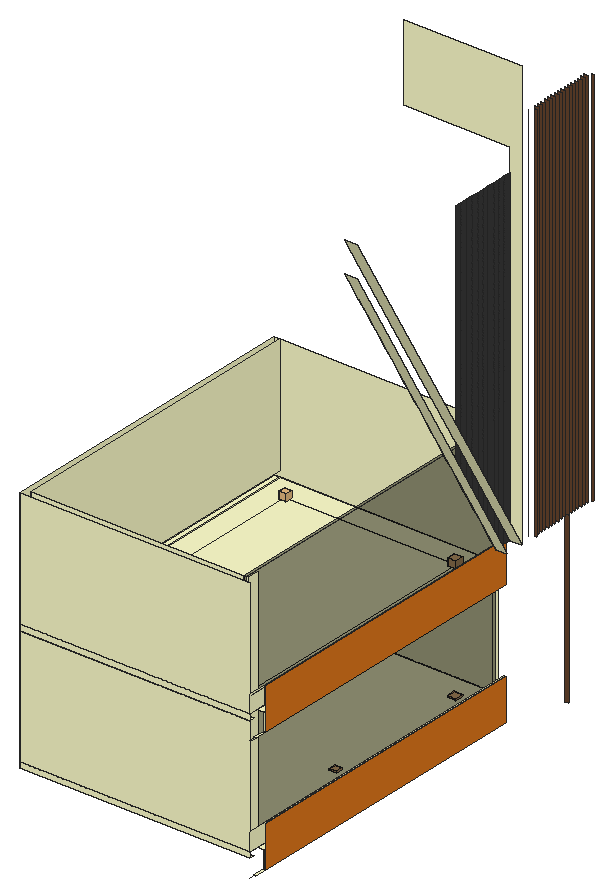
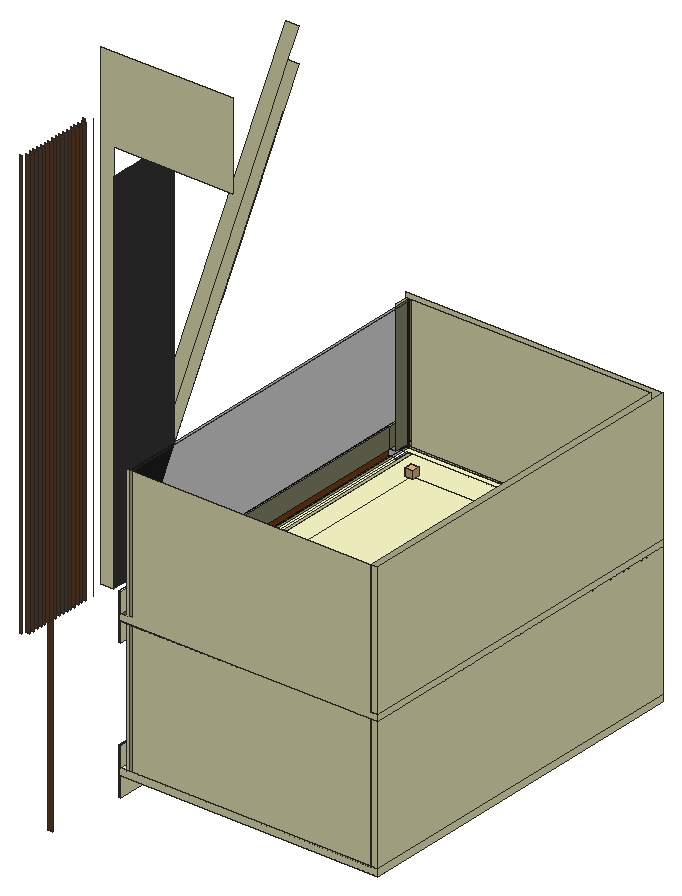
# SketchUp Ruby script. Lengths in inches.
U = 1.inch
M = Sketchup.active_model
def pt(a) = Geom::Point3d.new(a.map { |v| v * U })
def face(e, loops, mat)
  f = e.add_face(loops[0].map { |a| pt(a) })
  loops[1..].each { |l| e.add_face(l.map { |a| pt(a) }).erase! }
  f.material = f.back_material = mat if mat
  f
end
# faces: each face lists its corners as indices into pts; further lists are holes
def faces(e, pts, list, mat = nil) = list.each { |f| face(e, (f[0].is_a?(Array) ? f : [f]).map { |l| l.map { |i| pts[i] } }, mat) }
# xy, xz, yz: faces in a plane at the given z, y or x. An outline is a flat list of corners, or four numbers for a rectangle; further outlines are holes
def ring(l) = l.size == 4 ? [[l[0], l[1]], [l[2], l[1]], [l[2], l[3]], [l[0], l[3]]] : l.each_slice(2).to_a
def flat(e, list, mat, &to3) = list.each { |f| face(e, (f[0].is_a?(Array) ? f : [f]).map { |l| ring(l).map { |u, v| to3.(u, v) } }, mat) }
def xy(e, z, list, mat = nil) = flat(e, list, mat) { |x, y| [x, y, z] }
def xz(e, y, list, mat = nil) = flat(e, list, mat) { |x, z| [x, y, z] }
def yz(e, x, list, mat = nil) = flat(e, list, mat) { |y, z| [x, y, z] }
def lines(e, pts, list) = list.each { |a, b| e.add_line(pt(pts[a]), pt(pts[b])) }
# prism: a flat outline (further loops are holes) pulled along v
def prism(e, loops, v, mat = nil)
  f = face(e, loops, mat); d = Geom::Vector3d.new(v.map { |x| x * U })
  f.pushpull(f.normal.samedirection?(d) ? d.length : -d.length)
end
def box(e, o, s, mat = nil) = prism(e, [[o, [o[0] + s[0], o[1], o[2]], [o[0] + s[0], o[1] + s[1], o[2]], [o[0], o[1] + s[1], o[2]]]], [0, 0, s[2]], mat)
def at(x, y, z, deg = 0) = Geom::Transformation.translation(pt([x, y, z])) * Geom::Transformation.rotation(ORIGIN, Z_AXIS, deg.degrees)
def axes(o, x, y, z) = Geom::Transformation.new([*x, 0, *y, 0, *z, 0, *pt(o).to_a, 1])
def part(name) = M.definitions.add(name)
# library, detail: a bought-in or finely detailed component or shape, given as its bounding box
def library(name, o, s) = part(name).tap { |d| box(d.entities, o, s) }
def detail(e, o, s) = box(e.add_group.entities, o, s)
def put(e, d, t, mat = nil) = e.add_instance(d, t).tap { |i| i.material = mat if mat }
def group(e, t, mat = nil) = e.add_group.tap { |g| g.transformation = t; g.material = mat if mat }.entities
root = M.entities
M.materials.add("Brick_Common_Bond_2K").color = [226, 121, 29]
M.materials.add("E01_Mint_Frost").color = [255, 255, 204]
M.materials.add("Glass_Safety_01").color = [0, 0, 0]
M.materials["Glass_Safety_01"].alpha = 0.25
M.materials.add("M07_Charcoal_Gleam").color = [58, 58, 58]
M.materials.add("Wood_Veneer_15_1K").color = [103, 69, 45]
c1 = library("Sphere Light\#7",[-4.28,-4.28,-4.28],[8.56,8.56,8.56])
c2 = library("Sphere Light\#5",[-3.78,-3.78,-3.78],[7.56,7.56,7.56])
c3 = library("Sphere Light\#6",[-3.67,-3.67,-3.67],[7.34,7.34,7.34])
c4 = library("Sphere Light\#4",[-3.65,-3.65,-3.65],[7.3,7.3,7.3])
c5 = part("Group\#3")
box(c5.entities,[0,0,0],[3,318,120])
xy(root,240,[[469.07,81.71,471.07,93.71],[469.07,93.71,471.07,399.71]],"E01_Mint_Frost")
xy(root,258,[[235.07,75.71,469.07,81.71],[235.07,81.71,241.07,399.71],[[241.07,81.71,463.07,399.71],[439.07,101.71,440.11,101.85,441.07,102.25,441.9,102.89,442.54,103.71,442.9375,104.68,443.07,105.71,442.9375,106.75,442.54,107.71,441.9,108.54,441.07,109.18,440.11,109.58,439.07,109.71,439.07,371.72,440.02,371.83,441,372.21,441.84,372.82,442.49,373.64,442.91,374.59,443.07,375.625,442.96,376.66,442.58,377.64,441.96,378.48,441.15,379.13,440.19,379.55,439.16,379.71,438.125,379.6,437.15,379.22,436.31,378.6,435.65,377.79,435.23,376.83,435.07,375.8,435.08,375.71,269.05,375.71,269.0625,375.99,268.86,377.01,268.39,377.95,267.7,378.73,266.83,379.31,265.84,379.64,264.8,379.7,263.78,379.5,262.84,379.03,262.06,378.34,261.48,377.47,261.15,376.48,261.08,375.44,261.29,374.42,261.76,373.48,262.45,372.7,263.32,372.12,264.31,371.79,265.07,371.74,265.07,109.7,264.1875,109.61,263.21,109.25,262.35,108.65,261.6875,107.84,261.25,106.9,261.08,105.87,261.17,104.83,261.54,103.85,262.14,103,262.94,102.33,263.89,101.89,264.92,101.72,265.96,101.8125,266.94,102.18,267.79,102.78,268.46,103.58,268.9,104.53,269.07,105.5625,269.06,105.71,435.07,105.71,435.21,104.68,435.61,103.71,436.25,102.89,437.07,102.25,438.04,101.85]],[463.07,93.71,469.07,399.71],[269.06,105.71,268.97,106.6,268.61,107.58,268.01,108.43,267.2,109.1,266.25,109.54,265.23,109.71,265.07,109.7,265.07,371.74,265.35,371.72,266.37,371.93,267.31,372.4,268.09,373.09,268.67,373.96,269,374.95,269.05,375.71,435.08,375.71,435.1875,374.76,435.57,373.79,436.18,372.95,437,372.29,437.95,371.875,438.99,371.72,439.07,371.72,439.07,109.71,438.04,109.58,437.07,109.18,436.25,108.54,435.61,107.71,435.21,106.75,435.07,105.71]],"E01_Mint_Frost")
xy(root,261,[[439.07,101.71,438.04,101.85,437.07,102.25,436.25,102.89,435.61,103.71,435.21,104.68,435.07,105.71,435.21,106.75,435.61,107.71,436.25,108.54,437.07,109.18,438.04,109.58,439.07,109.71,440.11,109.58,441.07,109.18,441.9,108.54,442.54,107.71,442.9375,106.75,443.07,105.71,442.9375,104.68,442.54,103.71,441.9,102.89,441.07,102.25,440.11,101.85],[264.92,101.72,264.8,101.74,265.32,101.75],[264.8,101.74,264.29,101.83,263.78,101.94,263.31,102.16,262.85,102.41,262.45,102.74,262.07,103.1,261.77,103.52,261.49,103.96,261.3125,104.45,261.16,104.95,261.11,105.47,261.1,105.99,261.19,106.5,261.3,107.01,261.52,107.48,261.77,107.94,262.1,108.34,262.46,108.72,262.88,109.02,263.32,109.3,263.8125,109.48,264.3125,109.625,264.83,109.67,265.07,109.7,265.23,109.71,266.25,109.54,267.2,109.1,268.01,108.43,268.61,107.58,268.97,106.6,269.06,105.71,269.07,105.5625,269.05,105.4375,268.96,104.93,268.84,104.42,268.625,103.95,268.38,103.49,268.05,103.09,267.69,102.71,267.27,102.41,266.82,102.13,266.34,101.95,265.84,101.8,265.32,101.75],[265.84,101.8,266.34,101.95,265.96,101.8125],[264.29,101.83,263.89,101.89,263.78,101.94],
  [266.82,102.13,267.27,102.41,266.94,102.18],[263.31,102.16,262.94,102.33,262.85,102.41],[267.69,102.71,268.05,103.09,267.79,102.78],[262.45,102.74,262.14,103,262.07,103.1],[268.38,103.49,268.625,103.95,268.46,103.58],
  [261.77,103.52,261.54,103.85,261.49,103.96],[268.84,104.42,268.96,104.93,268.9,104.53],[261.3125,104.45,261.17,104.83,261.16,104.95],[261.11,105.47,261.08,105.87,261.1,105.99],[261.19,106.5,261.25,106.9,261.3,107.01],
  [261.52,107.48,261.6875,107.84,261.77,107.94],[262.1,108.34,262.35,108.65,262.46,108.72],[262.88,109.02,263.21,109.25,263.32,109.3],[263.8125,109.48,264.1875,109.61,264.3125,109.625],[265.35,371.72,265.07,371.74,264.31,371.79,263.32,372.12,262.45,372.7,261.76,373.48,261.29,374.42,261.08,375.44,261.15,376.48,261.48,377.47,262.06,378.34,262.84,379.03,263.78,379.5,264.8,379.7,265.84,379.64,266.83,379.31,267.7,378.73,268.39,377.95,268.86,377.01,269.0625,375.99,269.05,375.71,269,374.95,268.67,373.96,268.09,373.09,267.31,372.4,266.37,371.93],
  [438.99,371.72,437.95,371.875,437,372.29,436.18,372.95,435.57,373.79,435.1875,374.76,435.08,375.71,435.07,375.8,435.23,376.83,435.65,377.79,436.31,378.6,437.15,379.22,438.125,379.6,439.16,379.71,440.19,379.55,441.15,379.13,441.96,378.48,442.58,377.64,442.96,376.66,443.07,375.625,442.91,374.59,442.49,373.64,441.84,372.82,441,372.21,440.02,371.83,439.07,371.72]],"E01_Mint_Frost")
xy(root,264,[[235.07,75.71,469.07,75.71,469.07,93.71,463.07,93.71,463.07,81.71,241.07,81.71,241.07,399.71,235.07,399.71],[241.07,81.71,463.07,81.71,463.07,93.71,469.07,93.71,469.07,399.71,241.07,399.71]],"E01_Mint_Frost")
xy(root,282,[[469.07,93.71,471.07,399.71]],"E01_Mint_Frost")
xy(root,366,[[469.07,81.71,471.07,93.71],[469.07,93.71,471.07,399.71]],"E01_Mint_Frost")
xy(root,384,[[235.07,75.71,469.07,81.71],[235.07,81.71,241.07,399.71],[[241.07,81.71,463.07,399.71],[265.07,105.71,439.07,375.71]],[463.07,93.71,469.07,399.71],[265.07,105.71,439.07,375.71]],"E01_Mint_Frost")
xy(root,390,[[235.07,75.71,469.07,75.71,469.07,93.71,463.07,93.71,463.07,81.71,241.07,81.71,241.07,399.71,235.07,399.71]],"E01_Mint_Frost")
xy(root,408,[[469.07,93.71,471.07,399.71]],"E01_Mint_Frost")
xz(root,75.71,[[235.07,258,469.07,264],[235.07,264,469.07,384],[235.07,384,469.07,390],[235.07,390,469.07,510]],"E01_Mint_Frost")
xz(root,81.71,[[241.07,264,458.07,384],[461.07,264,463.07,384],[241.07,390,458.07,510],[461.07,390,463.07,510]],"E01_Mint_Frost")
xz(root,93.71,[[469.07,240,471.07,258]],"E01_Mint_Frost")
xz(root,371.72,[[438.99,258,439.07,261]],"E01_Mint_Frost")
xz(root,399.71,[[469.07,240,471.07,258],[235.07,258,471.07,264],[235.07,264,241.07,384],[241.07,264,463.07,384],[469.07,264,471.07,282],
  [469.07,366,471.07,384],[235.07,384,471.07,384,471.07,390,463.07,390,463.07,510,241.07,510,241.07,390,235.07,390],[235.07,390,241.07,510],[469.07,390,471.07,408],[475.07,408,487.07,408,487.07,846,367.07,846,367.07,768,475.07,768]],"E01_Mint_Frost")
xz(root,420,[[485.07,406.83,487.07,796.83]],"Wood_Veneer_15_1K")
xz(root,424.21,[[481.07,406.9,485.07,796.9]],"Wood_Veneer_15_1K")
xz(root,428.43,[[481.07,406.96,485.07,796.96]],"Wood_Veneer_15_1K")
xz(root,432.64,[[481.07,407.03,485.07,797.03]],"Wood_Veneer_15_1K")
xz(root,436.86,[[481.07,407.09,485.07,797.09]],"Wood_Veneer_15_1K")
xz(root,441.07,[[481.07,407.16,485.07,797.16]],"Wood_Veneer_15_1K")
xz(root,445.29,[[481.07,407.22,485.07,797.22]],"Wood_Veneer_15_1K")
xz(root,449.5,[[481.07,407.29,485.07,797.29]],"Wood_Veneer_15_1K")
xz(root,453.71,[[481.07,407.35,485.07,797.35]],"Wood_Veneer_15_1K")
xz(root,457.93,[[481.07,407.42,485.07,797.42]],"Wood_Veneer_15_1K")
xz(root,462.14,[[481.07,235.56,485.07,407.48],[481.07,407.48,485.07,797.48]],"Wood_Veneer_15_1K")
xz(root,466.36,[[481.07,407.55,485.07,797.55]],"Wood_Veneer_15_1K")
xz(root,470.57,[[481.07,407.61,485.07,797.61]],"Wood_Veneer_15_1K")
xz(root,474.79,[[481.07,407.68,485.07,797.68]],"Wood_Veneer_15_1K")
xz(root,479,[[481.07,407.74,485.07,797.74]],"Wood_Veneer_15_1K")
xz(root,483.21,[[481.07,407.81,485.07,797.81]],"Wood_Veneer_15_1K")
xz(root,487.43,[[481.07,407.87,485.07,797.87]],"Wood_Veneer_15_1K")
xz(root,491.64,[[485.07,407.94,487.07,797.94]],"Wood_Veneer_15_1K")
yz(root,235.07,[[75.71,258,399.71,264],[75.71,264,399.71,384],[75.71,384,399.71,390],[75.71,390,399.71,510]],"E01_Mint_Frost")
yz(root,241.07,[[81.71,264,399.71,384],[81.71,390,399.71,510]],"E01_Mint_Frost")
yz(root,463.07,[[81.71,264,93.71,384],[81.71,390,93.71,510]],"E01_Mint_Frost")
yz(root,469.07,[[93.71,240,399.71,258],[75.71,264,399.71,282],[93.71,366,399.71,384],[75.71,390,93.71,408],[93.71,390,399.71,408]],"E01_Mint_Frost")
yz(root,471.07,[[93.71,240,399.71,282],[93.71,366,399.71,408]],"Brick_Common_Bond_2K")
yz(root,475.07,[[381.71,408,386.03,408,386.03,744,379.18,744,379.18,412.43],[386.03,408,392.87,744],[392.87,408,399.71,744],[379.18,412.43,379.18,744,372.34,744,372.34,424.41],[372.34,424.41,372.34,744,365.49,744,365.49,436.39],
  [365.49,436.39,365.49,744,358.65,744,358.65,448.37],[358.65,448.37,358.65,744,351.8,744,351.8,460.35],[351.8,460.35,351.8,744,344.96,744,344.96,472.32],[344.96,472.32,344.96,744,338.11,744,338.11,484.3],[338.11,484.3,338.11,744,331.27,744,331.27,496.28]],"M07_Charcoal_Gleam")
p = [[264.92,101.72,258],[263.89,101.89,258],[263.89,101.89,261],[264.29,101.83,261],[264.8,101.74,261],[264.92,101.72,261],
  [265.96,101.8125,258],[265.32,101.75,261],[265.84,101.8,261],[265.96,101.8125,261],[439.07,101.71,258],[438.04,101.85,258],
  [438.04,101.85,261],[439.07,101.71,261],[440.11,101.85,258],[440.11,101.85,261],[266.94,102.18,258],[266.34,101.95,261],
  [266.82,102.13,261],[266.94,102.18,261],[262.94,102.33,258],[262.94,102.33,261],[263.31,102.16,261],[263.78,101.94,261],
  [437.07,102.25,258],[437.07,102.25,261],[441.07,102.25,258],[441.07,102.25,261],[267.79,102.78,258],[267.27,102.41,261],
  [267.69,102.71,261],[267.79,102.78,261],[262.14,103,258],[262.14,103,261],[262.45,102.74,261],[262.85,102.41,261],
  [436.25,102.89,258],[436.25,102.89,261],[441.9,102.89,258],[441.9,102.89,261],[268.46,103.58,258],[268.05,103.09,261],
  [268.38,103.49,261],[268.46,103.58,261],[435.61,103.71,258],[435.61,103.71,261],[442.54,103.71,258],[442.54,103.71,261],
  [261.54,103.85,258],[261.54,103.85,261],[261.77,103.52,261],[262.07,103.1,261],[268.9,104.53,258],[268.625,103.95,261],
  [268.84,104.42,261],[268.9,104.53,261],[435.21,104.68,258],[435.21,104.68,261],[442.9375,104.68,258],[442.9375,104.68,261],
  [261.17,104.83,258],[261.17,104.83,261],[261.3125,104.45,261],[261.49,103.96,261],[269.07,105.5625,258],[268.96,104.93,261],
  [269.05,105.4375,261],[269.07,105.5625,261],[435.07,105.71,258],[435.07,105.71,261],[443.07,105.71,258],[443.07,105.71,261],
  [261.08,105.87,258],[261.08,105.87,261],[261.11,105.47,261],[261.16,104.95,261],[269.06,105.71,258],[269.06,105.71,261],
  [268.97,106.6,258],[268.97,106.6,261],[435.21,106.75,258],[435.21,106.75,261],[442.9375,106.75,258],[442.9375,106.75,261],
  [261.25,106.9,258],[261.25,106.9,261],[261.19,106.5,261],[261.1,105.99,261],[268.61,107.58,258],[268.61,107.58,261],
  [435.61,107.71,258],[435.61,107.71,261],[442.54,107.71,258],[442.54,107.71,261],[261.6875,107.84,258],[261.6875,107.84,261],
  [261.52,107.48,261],[261.3,107.01,261],[268.01,108.43,258],[268.01,108.43,261],[436.25,108.54,258],[436.25,108.54,261],
  [441.9,108.54,258],[441.9,108.54,261],[262.35,108.65,258],[262.35,108.65,261],[262.1,108.34,261],[261.77,107.94,261],
  [267.2,109.1,258],[267.2,109.1,261],[437.07,109.18,258],[437.07,109.18,261],[441.07,109.18,258],[441.07,109.18,261],
  [263.21,109.25,258],[263.21,109.25,261],[262.88,109.02,261],[262.46,108.72,261],[266.25,109.54,258],[266.25,109.54,261],
  [438.04,109.58,258],[438.04,109.58,261],[440.11,109.58,258],[440.11,109.58,261],[264.1875,109.61,258],[264.1875,109.61,261],
  [263.8125,109.48,261],[263.32,109.3,261],[265.23,109.71,258],[265.23,109.71,261],[265.07,109.7,258],[265.07,109.7,261],
  [264.83,109.67,261],[264.3125,109.625,261],[439.07,109.71,258],[439.07,109.71,261],[265.07,371.74,258],[264.31,371.79,258],
  [264.31,371.79,261],[265.07,371.74,261],[265.35,371.72,258],[265.35,371.72,261],[266.37,371.93,258],[266.37,371.93,261],
  [438.99,371.72,258],[437.95,371.875,258],[437.95,371.875,261],[438.99,371.72,261],[440.02,371.83,258],[439.07,371.72,258],
  [439.07,371.72,261],[440.02,371.83,261],[263.32,372.12,258],[263.32,372.12,261],[441,372.21,258],[441,372.21,261],
  [267.31,372.4,258],[267.31,372.4,261],[437,372.29,258],[437,372.29,261],[262.45,372.7,258],[262.45,372.7,261],
  [441.84,372.82,258],[441.84,372.82,261],[436.18,372.95,258],[436.18,372.95,261],[268.09,373.09,258],[268.09,373.09,261],
  [261.76,373.48,258],[261.76,373.48,261],[442.49,373.64,258],[442.49,373.64,261],[435.57,373.79,258],[435.57,373.79,261],
  [268.67,373.96,258],[268.67,373.96,261],[261.29,374.42,258],[261.29,374.42,261],[442.91,374.59,258],[442.91,374.59,261],
  [435.1875,374.76,258],[435.1875,374.76,261],[269,374.95,258],[269,374.95,261],[261.08,375.44,258],[261.08,375.44,261],
  [443.07,375.625,258],[443.07,375.625,261],[435.08,375.71,258],[435.08,375.71,261],[269.05,375.71,258],[269.05,375.71,261],
  [261.15,376.48,258],[261.15,376.48,261],[442.96,376.66,258],[442.96,376.66,261],[269.0625,375.99,258],[269.0625,375.99,261],
  [435.07,375.8,258],[435.07,375.8,261],[435.23,376.83,258],[435.23,376.83,261],[268.86,377.01,258],[268.86,377.01,261],
  [261.48,377.47,258],[261.48,377.47,261],[442.58,377.64,258],[442.58,377.64,261],[435.65,377.79,258],[435.65,377.79,261],
  [268.39,377.95,258],[268.39,377.95,261],[262.06,378.34,258],[262.06,378.34,261],[441.96,378.48,258],[441.96,378.48,261],
  [436.31,378.6,258],[436.31,378.6,261],[267.7,378.73,258],[267.7,378.73,261],[262.84,379.03,258],[262.84,379.03,261],
  [441.15,379.13,258],[441.15,379.13,261],[437.15,379.22,258],[437.15,379.22,261],[266.83,379.31,258],[266.83,379.31,261],
  [263.78,379.5,258],[263.78,379.5,261],[440.19,379.55,258],[440.19,379.55,261],[438.125,379.6,258],[438.125,379.6,261],
  [265.84,379.64,258],[265.84,379.64,261],[264.8,379.7,258],[264.8,379.7,261],[439.16,379.71,258],[439.16,379.71,261],
  [487.07,381.71,408],[487.07,189.71,744],[475.19,189.71,744],[475.07,189.71,744],[475.07,194.38,735.84],[475.07,201.22,723.86],
  [475.07,208.07,711.88],[475.07,214.91,699.9],[475.07,221.76,687.93],[475.07,228.6,675.95],[475.07,235.45,663.97],[475.07,242.29,651.99],
  [475.07,249.13,640.01],[475.07,255.98,628.04],[475.07,262.82,616.06],[475.07,269.67,604.08],[475.07,276.51,592.1],[475.07,283.36,580.125],
  [475.07,290.2,568.15],[475.07,297.05,556.17],[475.07,303.89,544.19],[475.07,310.74,532.21],[475.07,317.58,520.23],[475.07,324.42,508.26],
  [475.07,331.27,496.28],[475.07,338.11,484.3],[475.07,344.96,472.32],[475.07,351.8,460.35],[475.07,358.65,448.37],[475.07,365.49,436.39],
  [475.07,372.34,424.41],[475.07,379.18,412.43],[475.07,381.71,408],[487.07,189.71,775],[487.07,399.71,408],[475.19,399.71,408],
  [475.19,207.71,743.54],[475.19,207.45,744],[475.19,189.71,775],[481.07,415.79,796.77],[481.07,415.79,406.77],[475.19,207.71,712.5],
  [475.09,380.51,410.1],[469.07,81.71,240],[469.07,75.71,240],[469.07,81.71,366],[469.07,75.71,366],[463.07,399.71,390],
  [463.07,153.71,390],[471.07,75.71,408],[471.07,93.71,408],[471.07,81.71,366],[471.07,75.71,366],[463.07,399.71,264],
  [463.07,153.71,264],[469.07,93.71,384],[471.07,93.71,384],[261.98,103.18,387],[262.74,102.47,387],[265.07,109.68,387],
  [264.43,109.66,387],[263.43,109.36,387],[262.54,108.8125,387],[261.83,108.05,387],[261.33,107.13,387],[261.09,106.11,387],
  [261.125,105.07,387],[261.43,104.07,387],[263.66,101.97,387],[264.67,101.73,387],[265.72,101.77,387],[266.72,102.07,387],
  [267.6,102.62,387],[268.32,103.38,387],[268.81,104.3,387],[269.05,105.3125,387],[269.04,105.71,387],[266.72,102.07,261],
  [265.07,109.68,261],[264.43,109.66,261],[263.43,109.36,261],[262.54,108.8125,261],[261.83,108.05,261],[261.33,107.13,261],
  [261.09,106.11,261],[261.125,105.07,261],[261.43,104.07,261],[261.98,103.18,261],[262.74,102.47,261],[263.66,101.97,261],
  [264.67,101.73,261],[265.72,101.77,261],[267.6,102.62,261],[268.32,103.38,261],[268.81,104.3,261],[269.05,105.3125,261],
  [269.04,105.71,261],[267.78,225.56,258.53],[266.98,226.23,258.53],[268.83,222.84,258.53],[268.75,223.73,258.53],[268.39,224.71,258.53],
  [266.03,226.66,258.53],[265,226.84,258.53],[264.85,226.82,258.53]]
faces(root,p,[[0,1,2,3,4,5],[6,0,5,7,8,9],[10,11,12,13],[14,10,13,15],[16,6,9,17,18,19],[1,20,21,22,23,2],[11,24,25,12],[26,14,15,27],
  [28,16,19,29,30,31],[20,32,33,34,35,21],[24,36,37,25],[38,26,27,39],[40,28,31,41,42,43],[36,44,45,37],[46,38,39,47],[32,48,49,50,51,33],
  [52,40,43,53,54,55],[44,56,57,45],[58,46,47,59],[48,60,61,62,63,49],[64,52,55,65,66,67],[56,68,69,57],[70,58,59,71],[60,72,73,74,75,61],
  [76,64,67,77],[78,76,77,79],[68,80,81,69],[82,70,71,83],[72,84,85,86,87,73],[88,78,79,89],[80,90,91,81],[92,82,83,93],
  [84,94,95,96,97,85],[98,88,89,99],[90,100,101,91],[102,92,93,103],[94,104,105,106,107,95],[108,98,99,109],[100,110,111,101],[112,102,103,113],
  [104,114,115,116,117,105],[118,108,109,119],[110,120,121,111],[122,112,113,123],[114,124,125,126,127,115],[128,118,119,129],[124,130,131,132,133,125],[120,134,135,121],
  [134,122,123,135],[130,128,129,131],[136,137,138,139],[140,136,139,141],[142,140,141,143],[144,145,146,147],[148,149,150,151],[137,152,153,138],
  [154,148,151,155],[156,142,143,157],[145,158,159,146],[152,160,161,153],[162,154,155,163],[158,164,165,159],[166,156,157,167],[160,168,169,161],
  [170,162,163,171],[164,172,173,165],[174,166,167,175],[168,176,177,169],[178,170,171,179],[172,180,181,173],[182,174,175,183],[176,184,185,177],
  [186,178,179,187],[180,188,189,181],[190,182,183,191],[184,192,193,185],[194,186,187,195],[196,190,191,197],[188,198,199,189],[198,200,201,199],
  [202,196,197,203],[192,204,205,193],[206,194,195,207],[200,208,209,201],[210,202,203,211],[204,212,213,205],[214,206,207,215],[208,216,217,209],
  [218,210,211,219],[212,220,221,213],[222,214,215,223],[216,224,225,217],[226,218,219,227],[220,228,229,221],[230,222,223,231],[224,232,233,225],
  [234,226,227,235],[228,236,237,229],[236,234,235,237],[232,238,239,233],[238,230,231,239],[240,241,242,243,244,245,246,247,248,249,250,251,252,253,254,255,256,257,258,259,260,261,262,263,264,265,266,267,268,269,270,271,272],[273,274,275,276,277,278]],"E01_Mint_Frost")
lines(root,p,[[279,280],[281,282],[283,284],[285,286],[287,288],[289,290],[291,292],[293,294],[295,296],[297,298],[299,300],[300,301],
  [301,302],[302,303],[303,304],[304,305],[305,306],[306,307],[307,297],[298,308],[308,309],[309,310],[310,311],[311,312],
  [312,313],[313,314],[314,315],[315,316],[317,18],[318,132],[319,133],[320,127],[321,117],[322,107],[323,97],[324,87],
  [325,75],[326,63],[327,51],[328,35],[329,23],[330,4],[331,8],[332,30],[333,42],[334,54],[335,66],[132,319],
  [126,320],[116,321],[106,322],[96,323],[86,324],[74,325],[7,331],[66,336],[29,332],[62,326],[50,327],[34,328],
  [22,329],[3,330],[17,317],[41,333],[53,334],[65,335],[337,338],[339,340],[340,341],[341,337],[338,342],[342,343],
  [343,344]])
put(root,c1,at(439.21,375.11,261),"E01_Mint_Frost")
put(root,c2,at(265.13,106.05,261),"E01_Mint_Frost")
put(root,c3,at(265.53,375.54,261),"E01_Mint_Frost")
put(root,c4,at(439.3,105.8,261),"E01_Mint_Frost")
put(root,c2,at(264.91,223.18,261.53),"E01_Mint_Frost")
put(root,c4,at(439.07,222.92,261.53),"E01_Mint_Frost")
put(root,c5,at(458.07,81.71,264),"Glass_Safety_01")
put(root,c1,at(439.21,375.11,387),"E01_Mint_Frost")
put(root,c2,at(265.13,106.05,387),"E01_Mint_Frost")
put(root,c3,at(265.53,375.54,387),"E01_Mint_Frost")
put(root,c4,at(439.3,105.8,387),"E01_Mint_Frost")
put(root,c5,at(458.07,81.71,390),"Glass_Safety_01")
